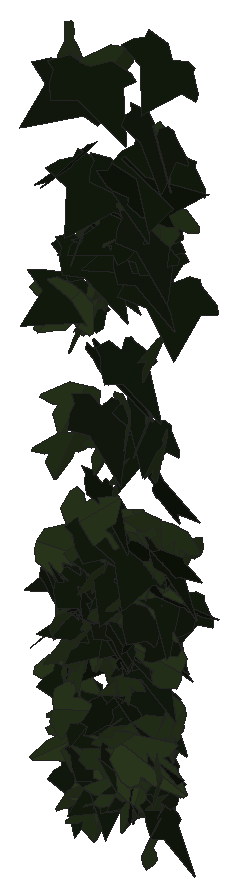
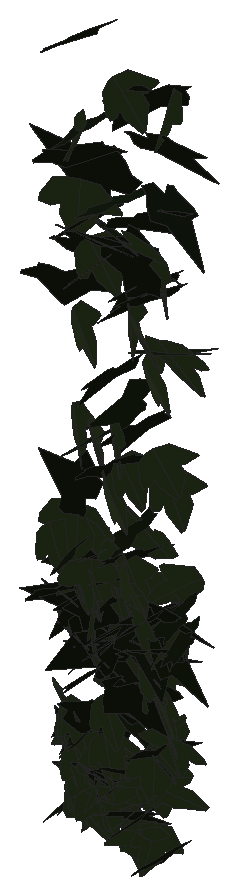
# SketchUp Ruby script. Lengths in inches.
U = 1.inch
M = Sketchup.active_model
def pt(a) = Geom::Point3d.new(a.map { |v| v * U })
def face(e, loops, mat)
  f = e.add_face(loops[0].map { |a| pt(a) })
  loops[1..].each { |l| e.add_face(l.map { |a| pt(a) }).erase! }
  f.material = f.back_material = mat if mat
  f
end
# faces: each face lists its corners as indices into pts; further lists are holes
def faces(e, pts, list, mat = nil) = list.each { |f| face(e, (f[0].is_a?(Array) ? f : [f]).map { |l| l.map { |i| pts[i] } }, mat) }
# xy, xz, yz: faces in a plane at the given z, y or x. An outline is a flat list of corners, or four numbers for a rectangle; further outlines are holes
def ring(l) = l.size == 4 ? [[l[0], l[1]], [l[2], l[1]], [l[2], l[3]], [l[0], l[3]]] : l.each_slice(2).to_a
def flat(e, list, mat, &to3) = list.each { |f| face(e, (f[0].is_a?(Array) ? f : [f]).map { |l| ring(l).map { |u, v| to3.(u, v) } }, mat) }
def xy(e, z, list, mat = nil) = flat(e, list, mat) { |x, y| [x, y, z] }
def xz(e, y, list, mat = nil) = flat(e, list, mat) { |x, z| [x, y, z] }
def yz(e, x, list, mat = nil) = flat(e, list, mat) { |y, z| [x, y, z] }
def lines(e, pts, list) = list.each { |a, b| e.add_line(pt(pts[a]), pt(pts[b])) }
# prism: a flat outline (further loops are holes) pulled along v
def prism(e, loops, v, mat = nil)
  f = face(e, loops, mat); d = Geom::Vector3d.new(v.map { |x| x * U })
  f.pushpull(f.normal.samedirection?(d) ? d.length : -d.length)
end
def box(e, o, s, mat = nil) = prism(e, [[o, [o[0] + s[0], o[1], o[2]], [o[0] + s[0], o[1] + s[1], o[2]], [o[0], o[1] + s[1], o[2]]]], [0, 0, s[2]], mat)
def at(x, y, z, deg = 0) = Geom::Transformation.translation(pt([x, y, z])) * Geom::Transformation.rotation(ORIGIN, Z_AXIS, deg.degrees)
def axes(o, x, y, z) = Geom::Transformation.new([*x, 0, *y, 0, *z, 0, *pt(o).to_a, 1])
def part(name) = M.definitions.add(name)
# library, detail: a bought-in or finely detailed component or shape, given as its bounding box
def library(name, o, s) = part(name).tap { |d| box(d.entities, o, s) }
def detail(e, o, s) = box(e.add_group.entities, o, s)
def put(e, d, t, mat = nil) = e.add_instance(d, t).tap { |i| i.material = mat if mat }
def group(e, t, mat = nil) = e.add_group.tap { |g| g.transformation = t; g.material = mat if mat }.entities
root = M.entities
M.materials.add("1026 AP 7946 SUNNY SIDE UP").color = [254, 231, 186]
M.materials.add("efeu1").color = [18, 25, 13]
M.materials.add("efeu2").color = [43, 57, 29]
c1 = part("ivyleaf_10")
p = [[0,0.5,-0.03],[-0.0625,2.02,-0.43],[-0.19,2.01,-0.46],[-0.54,1.05,-0.29],[-0.52,0.625,-0.18],[-0.83,0.76,-0.28],
  [-1.16,0.64,-0.33],[-1.15,0.33,-0.24],[-0.77,-0.39,0.02],[-0.3,-0.51,0.16],[0.04,-0.48,0.23],[-0.02,2.01,-0.4375],
  [-0.06,2.01,-0.43],[0.04,-0.49,0.23],[0.67,-0.49,0.14],[1.38,0.36,-0.2],[1.375,0.51,-0.24],[0.81,0.65,-0.19],
  [0.62,0.59,-0.15],[0.6,1.09,-0.28],[0.5,1.23,-0.31]]
faces(c1.entities,p,[[0,1,2,3,4,5,6,7,8,9,10],[11,12,0,13,14,15,16,17,18,19,20]],"efeu2")
c2 = part("ivyleaf_9")
p = [[1.54,2.16,1.25],[1.36,2.04,1.19],[-0.21,0.99,0.68],[-0.71,1.11,0.82],[-0.85,0.86,0.67],[-0.8,0.17,0.21],
  [-0.9,-0.01,0.1],[-0.67,-0.16,-0.02],[-0.08,-0.08,-0.05],[-0.03,-0.6,-0.4],[0.65,-0.88,-0.66],[0.83,-0.6,-0.49],
  [1.29,-0.42,-0.43],[1.8125,-0.07,-0.26],[1.21,0.44,0.15]]
faces(c2.entities,p,[[0,1,2,3,4,5,6,7,8,9,10,11,12,13,14]],"efeu1")
put(root,c1,axes([114.93,212.78,269.58],[0.41949,-0.00807,0.009],[0.01252,-0.02601,-0.27383],[0.01397,0.26566,-0.02496]),"1026 AP 7946 SUNNY SIDE UP")
put(root,c2,axes([114.86,212.53,271.03],[0.28826,-0.17994,-0.10556],[-0.0991,0.08044,-0.26386],[0.30931,0.19346,0.01384]),"1026 AP 7946 SUNNY SIDE UP")
put(root,c1,axes([115.09,212.77,270],[0.17426,-0.24249,-0.06948],[-0.06111,0.05481,-0.27406],[0.39044,0.1168,-0.01188]),"1026 AP 7946 SUNNY SIDE UP")
put(root,c1,axes([115.125,212.57,275.14],[0.43229,-0.08407,-0.10623],[-0.16878,-0.00212,-0.2944],[0.12262,0.29345,-0.03071]),"1026 AP 7946 SUNNY SIDE UP")
put(root,c1,axes([115.11,212.79,273.64],[-0.17544,-0.24056,0.1207],[0.00506,-0.12957,-0.26854],[0.42165,-0.09854,0.05344]),"1026 AP 7946 SUNNY SIDE UP")
put(root,c1,axes([115.03,212.61,278.78],[0.08865,-0.23721,-0.20622],[0.08034,0.20646,-0.23762],[0.48001,0.00925,0.07785]),"1026 AP 7946 SUNNY SIDE UP")
put(root,c2,axes([115.26,212.74,278.21],[-0.47065,-0.05058,0.01626],[-0.01884,-0.02524,-0.31199],[0.08129,-0.29868,0.0218]),"1026 AP 7946 SUNNY SIDE UP")
put(root,c2,axes([115.28,212.43,277.23],[-0.16105,0.28001,-0.03059],[0.00343,-0.03249,-0.30721],[-0.44302,-0.10205,0.00874]),"1026 AP 7946 SUNNY SIDE UP")
put(root,c1,axes([115.25,212.62,268.78],[0.1942,0.10053,-0.22778],[-0.29186,-0.1219,-0.1642],[-0.24758,0.22256,0.0149]),"1026 AP 7946 SUNNY SIDE UP")
put(root,c2,axes([115.22,212.72,275.13],[-0.38554,-0.12197,0.11628],[-0.03425,-0.17684,-0.24514],[0.25981,-0.20431,0.14024]),"1026 AP 7946 SUNNY SIDE UP")
put(root,c1,axes([115.18,212.5,273.13],[-0.14112,-0.27861,0.04935],[-0.01071,-0.04977,-0.30171],[0.44482,-0.08959,0.00839]),"1026 AP 7946 SUNNY SIDE UP")
put(root,c2,axes([115.05,212.93,267.92],[-0.06722,-0.24107,0.08265],[-0.01766,-0.08087,-0.25268],[0.39979,-0.04411,0.00273]),"1026 AP 7946 SUNNY SIDE UP")
put(root,c2,axes([114.93,212.54,271.35],[0.26419,-0.22109,-0.04019],[-0.04297,0.02665,-0.28586],[0.35005,0.17014,-0.00476]),"1026 AP 7946 SUNNY SIDE UP")
put(root,c2,axes([115.32,212.43,270.72],[-0.20392,0.2082,-0.12161],[0.06496,-0.11412,-0.25227],[-0.37161,-0.1342,0.02263]),"1026 AP 7946 SUNNY SIDE UP")
put(root,c1,axes([115.06,212.27,271.65],[0.05061,0.12629,0.26446],[0.09311,0.24905,-0.13279],[-0.43908,0.06737,0.00232]),"1026 AP 7946 SUNNY SIDE UP")
put(root,c2,axes([115.14,212.78,269.42],[-0.15404,-0.24708,0.01632],[0.00685,-0.02026,-0.27368],[0.3894,-0.09738,0.01127]),"1026 AP 7946 SUNNY SIDE UP")
put(root,c1,axes([115.22,212.82,274.88],[0.15842,-0.26962,0.06208],[0.01339,-0.0627,-0.29655],[0.43474,0.10018,-0.01349]),"1026 AP 7946 SUNNY SIDE UP")
put(root,c1,axes([115.28,212.51,269.99],[0.25029,-0.19239,-0.11752],[-0.08352,0.10212,-0.25564],[0.34074,0.16635,0.02366]),"1026 AP 7946 SUNNY SIDE UP")
put(root,c1,axes([115.26,212.71,269.17],[-0.26627,-0.20241,-0.0173],[0.02633,0.00637,-0.27169],[0.31813,-0.16994,0.00801]),"1026 AP 7946 SUNNY SIDE UP")
put(root,c1,axes([115.21,212.26,270.75],[-0.01818,-0.08253,-0.2877],[0.08763,0.27322,-0.08411],[0.44871,-0.0567,0.00477]),"1026 AP 7946 SUNNY SIDE UP")
put(root,c2,axes([115.54,212.63,271.34],[-0.42803,0.02994,0.05849],[-0.09319,-0.02411,-0.28059],[-0.03816,-0.27699,0.02909]),"1026 AP 7946 SUNNY SIDE UP")
put(root,c1,axes([115.36,212.48,276.22],[0.17653,-0.2613,-0.09098],[-0.02078,0.08854,-0.2916],[0.43246,0.11092,0.02312]),"1026 AP 7946 SUNNY SIDE UP")
put(root,c1,axes([115.32,212.61,268.05],[-0.15118,-0.22286,-0.11078],[0.0885,0.09125,-0.24908],[0.378,-0.1105,0.01401]),"1026 AP 7946 SUNNY SIDE UP")
put(root,c2,axes([115.47,212.55,270.84],[0.04089,0.26936,-0.00898],[-0.04255,-0.00763,-0.27752],[-0.4217,0.02689,0.02713]),"1026 AP 7946 SUNNY SIDE UP")
put(root,c1,axes([115.28,212.2,269.41],[0.03883,-0.11464,-0.26362],[0.18173,0.23753,-0.097],[0.40068,-0.09663,0.06954]),"1026 AP 7946 SUNNY SIDE UP")
put(root,c1,axes([115.41,212.33,270.33],[-0.14821,-0.25404,-0.09716],[0.05128,0.08696,-0.27864],[0.42221,-0.09974,-0.00026]),"1026 AP 7946 SUNNY SIDE UP")
put(root,c2,axes([115.55,212.67,270.13],[0.12324,0.15952,-0.2085],[-0.12133,-0.1883,-0.18397],[-0.38779,0.10961,-0.0087]),"1026 AP 7946 SUNNY SIDE UP")
put(root,c2,axes([115.68,212.72,270.5625],[-0.328,-0.06195,0.16458],[-0.19106,-0.12472,-0.21352],[0.19071,-0.2315,0.06915]),"1026 AP 7946 SUNNY SIDE UP")
put(root,c1,axes([115.18,212.83,276.52],[-0.16762,-0.00929,-0.29057],[0.36942,-0.16987,-0.08672],[-0.24569,-0.24907,0.06785]),"1026 AP 7946 SUNNY SIDE UP")
put(root,c1,axes([115.43,212.76,268.07],[0.2581,0.20013,-0.04493],[-0.0206,-0.04697,-0.26618],[-0.3218,0.16353,-0.019]),"1026 AP 7946 SUNNY SIDE UP")
put(root,c1,axes([115.43,212.76,275.31],[0.29729,-0.20461,0.10986],[0.0809,-0.09853,-0.28622],[0.35454,0.19406,-0.02681]),"1026 AP 7946 SUNNY SIDE UP")
put(root,c2,axes([115.34,212.65,268.58],[0.16106,-0.22662,-0.09419],[-0.03735,0.08804,-0.2553],[0.38167,0.10425,0.01476]),"1026 AP 7946 SUNNY SIDE UP")
put(root,c1,axes([115.5625,212.79,271.83],[0.0037,-0.28086,0.03917],[-0.00028,-0.03962,-0.28958],[0.44599,0.0023,-0.00051]),"1026 AP 7946 SUNNY SIDE UP")
put(root,c2,axes([115.29,212.66,275.9375],[0.14096,-0.25137,-0.15367],[0.0471,0.16169,-0.26373],[0.45604,0.061,0.07474]),"1026 AP 7946 SUNNY SIDE UP")
put(root,c1,axes([115.4,212.77,270.41],[0.37382,-0.1097,0.09198],[0.12465,-0.04274,-0.26993],[0.18493,0.25055,-0.00398]),"1026 AP 7946 SUNNY SIDE UP")
put(root,c2,axes([115.41,212.75,271.16],[-0.04881,-0.27369,0.06293],[-0.00309,-0.06281,-0.28408],[0.44147,-0.0307,0.00497]),"1026 AP 7946 SUNNY SIDE UP")
put(root,c2,axes([115.56,212.7,276.96],[-0.29439,-0.23287,0.05993],[-0.01984,-0.06579,-0.30656],[0.3774,-0.1851,0.03063]),"1026 AP 7946 SUNNY SIDE UP")
put(root,c1,axes([115.59,212.7,271.17],[0.31452,-0.18049,-0.07948],[-0.06424,0.06797,-0.27621],[0.30124,0.20294,0.02409]),"1026 AP 7946 SUNNY SIDE UP")
put(root,c2,axes([115.4,212.48,271.21],[0.03551,-0.24407,-0.1405],[0.01794,0.13613,-0.25079],[0.4382,0.01421,0.02166]),"1026 AP 7946 SUNNY SIDE UP")
put(root,c1,axes([115.64,212.51,267.94],[-0.14285,-0.25031,-0.01871],[0.02269,0.01256,-0.27409],[0.39382,-0.09152,0.00901]),"1026 AP 7946 SUNNY SIDE UP")
put(root,c1,axes([115.59,212.74,275.6],[0.11293,-0.28849,-0.03148],[0.06893,0.04026,-0.30131],[0.45065,0.06614,0.05397]),"1026 AP 7946 SUNNY SIDE UP")
put(root,c1,axes([115.38,212.54,268.69],[-0.21123,-0.05842,-0.22803],[0.34761,0.03211,-0.14698],[0.09158,-0.25664,0.03192]),"1026 AP 7946 SUNNY SIDE UP")
put(root,c2,axes([115.875,212.45,269.48],[-0.2352,0.22892,0.06602],[-0.06689,0.04715,-0.28127],[-0.36721,-0.15522,0.00895]),"1026 AP 7946 SUNNY SIDE UP")
put(root,c2,axes([115.44,212.58,275.99],[0.06549,-0.28884,-0.09893],[0.034,0.09785,-0.29806],[0.4766,0.03271,0.03486]),"1026 AP 7946 SUNNY SIDE UP")
put(root,c1,axes([115.69,212.74,273.29],[-0.04208,-0.27444,0.08002],[0.00642,-0.07994,-0.28429],[0.44911,-0.02457,0.01156]),"1026 AP 7946 SUNNY SIDE UP")
put(root,c1,axes([115.74,212.77,278.8],[-0.10948,-0.27775,0.11201],[-0.02523,-0.10962,-0.29544],[0.46924,-0.0707,0.01025]),"1026 AP 7946 SUNNY SIDE UP")
put(root,c2,axes([115.57,212.76,268.2],[-0.02878,-0.25262,0.07261],[-0.014,-0.07146,-0.26132],[0.41277,-0.02004,-0.0038]),"1026 AP 7946 SUNNY SIDE UP")
put(root,c1,axes([115.67,212.51,271.62],[-0.40683,-0.10944,-0.04361],[0.0781,-0.01094,-0.28791],[0.16677,-0.26184,0.02845]),"1026 AP 7946 SUNNY SIDE UP")
put(root,c2,axes([115.3,212.81,276.43],[0.17542,-0.00496,-0.29026],[0.43514,0.05895,0.11217],[0.08338,-0.29722,0.02529]),"1026 AP 7946 SUNNY SIDE UP")
put(root,c1,axes([115.73,212.47,271.46],[-0.02201,-0.2661,-0.09388],[0.01474,0.08924,-0.27396],[0.44127,-0.01625,0.00447]),"1026 AP 7946 SUNNY SIDE UP")
put(root,c2,axes([115.49,212.79,272.4375],[0.1315,-0.26089,0.07762],[0.02042,-0.07645,-0.28248],[0.42715,0.08397,-0.01039]),"1026 AP 7946 SUNNY SIDE UP")
put(root,c2,axes([115.53,212.4375,278.68],[-0.04491,-0.26333,-0.18299],[0.0668,0.17207,-0.2711],[0.49364,-0.04724,0.02004]),"1026 AP 7946 SUNNY SIDE UP")
put(root,c2,axes([115.47,212.75,274.37],[0.32076,-0.2051,-0.04694],[-0.02864,0.04438,-0.29716],[0.32872,0.20399,0.01992]),"1026 AP 7946 SUNNY SIDE UP")
put(root,c1,axes([115.45,212.4,272.09],[0.35817,-0.08196,-0.17884],[0.26975,-0.03239,0.24813],[-0.134,-0.28427,0.02147]),"1026 AP 7946 SUNNY SIDE UP")
put(root,c2,axes([115.87,212.66,270.63],[-0.39784,-0.09277,0.02579],[-0.02289,-0.03417,-0.27643],[0.14957,-0.252,0.02629]),"1026 AP 7946 SUNNY SIDE UP")
put(root,c2,axes([115.86,212.79,268.23],[-0.33661,-0.11831,0.10196],[-0.07977,-0.10703,-0.24381],[0.22977,-0.21048,0.06473]),"1026 AP 7946 SUNNY SIDE UP")
put(root,c1,axes([115.51,212.83,271.73],[0.23915,-0.05706,0.25343],[0.34876,-0.10791,-0.16746],[0.19089,0.26864,-0.01154]),"1026 AP 7946 SUNNY SIDE UP")
put(root,c2,axes([115.625,212.57,270.89],[0.13223,-0.26859,0.01094],[-0.00802,-0.01432,-0.28988],[0.42269,0.08375,-0.00893]),"1026 AP 7946 SUNNY SIDE UP")
put(root,c2,axes([115.72,212.77,268.91],[-0.17519,-0.23128,-0.06134],[0.1205,0.02615,-0.25789],[0.35513,-0.12296,0.05724]),"1026 AP 7946 SUNNY SIDE UP")
put(root,c1,axes([115.9,212.61,268.28],[-0.1383,-0.21603,0.12673],[-0.0209,-0.12749,-0.23883],[0.3913,-0.08317,0.03203]),"1026 AP 7946 SUNNY SIDE UP")
put(root,c1,axes([115.85,212.57,270.05],[-0.40292,0.09737,-0.02463],[0.02107,-0.03328,-0.28129],[-0.15645,-0.25525,0.02555]),"1026 AP 7946 SUNNY SIDE UP")
put(root,c2,axes([115.61,212.53,272.02],[0.13818,-0.23822,-0.15891],[0.06674,0.16938,-0.24574],[0.44007,0.04911,0.08717]),"1026 AP 7946 SUNNY SIDE UP")
put(root,c1,axes([115.78,212.52,268.73],[-0.35601,-0.07509,-0.10666],[0.1711,-0.00409,-0.24311],[0.10466,-0.24875,0.03461]),"1026 AP 7946 SUNNY SIDE UP")
put(root,c1,axes([115.89,212.78,272.9],[0.1088,-0.27306,0.05565],[0.02304,-0.05361,-0.29051],[0.43755,0.07072,0.00146]),"1026 AP 7946 SUNNY SIDE UP")
put(root,c2,axes([115.74,212.47,273.78],[0.00151,-0.29732,-0.06051],[-0.01785,0.05698,-0.30576],[0.4757,0.00308,-0.01128]),"1026 AP 7946 SUNNY SIDE UP")
put(root,c2,axes([116.16,212.51,276.51],[-0.42561,0.12949,-0.00205],[-0.03625,-0.05439,-0.3034],[-0.2004,-0.26517,0.05924]),"1026 AP 7946 SUNNY SIDE UP")
put(root,c1,axes([115.95,212.79,269.76],[-0.1104,-0.26402,0.02196],[0.00644,-0.02468,-0.28139],[0.41664,-0.06958,0.01017]),"1026 AP 7946 SUNNY SIDE UP")
put(root,c2,axes([115.85,212.91,273.36],[-0.15453,-0.26404,0.02867],[0.00006,-0.03129,-0.2902],[0.41772,-0.09767,0.01065]),"1026 AP 7946 SUNNY SIDE UP")
put(root,c1,axes([115.98,212.625,273.73],[0.2127,-0.20317,-0.16155],[-0.06119,0.1577,-0.24594],[0.39777,0.1329,0.04855]),"1026 AP 7946 SUNNY SIDE UP")
put(root,c1,axes([115.98,212.76,269.1875],[-0.12488,-0.25534,-0.00944],[0.00521,0.00705,-0.27544],[0.40165,-0.07948,0.00064]),"1026 AP 7946 SUNNY SIDE UP")
put(root,c1,axes([115.88,212.76,268.52],[0.32865,0.16156,-0.01929],[-0.00114,-0.03106,-0.2712],[-0.25591,0.20762,-0.02358]),"1026 AP 7946 SUNNY SIDE UP")
put(root,c2,axes([115.95,212.65,271.5],[-0.23666,-0.2353,0.02336],[-0.00264,-0.0274,-0.28758],[0.3719,-0.14993,0.01283]),"1026 AP 7946 SUNNY SIDE UP")
put(root,c1,axes([116.03,212.72,268.98],[-0.29337,-0.19053,0.01532],[0.00226,-0.02369,-0.27426],[0.30064,-0.18575,0.01701]),"1026 AP 7946 SUNNY SIDE UP")
put(root,c1,axes([115.95,212.375,271],[-0.17426,-0.22889,-0.12487],[0.10375,0.10109,-0.261],[0.39283,-0.12823,0.01354]),"1026 AP 7946 SUNNY SIDE UP")
put(root,c2,axes([115.61,212.6,270.44],[0.26033,-0.13659,0.17653],[0.26101,-0.06347,-0.21675],[0.2264,0.23024,0.0469]),"1026 AP 7946 SUNNY SIDE UP")
put(root,c1,axes([116.07,212.84,268.41],[-0.24861,-0.19558,0.07864],[-0.04434,-0.0763,-0.25827],[0.32778,-0.15866,0.02471]),"1026 AP 7946 SUNNY SIDE UP")
put(root,c2,axes([115.83,212.71,268.7],[0.09572,-0.25027,0.07398],[0.0087,-0.07395,-0.2655],[0.40993,0.06001,-0.01164]),"1026 AP 7946 SUNNY SIDE UP")
put(root,c2,axes([116.04,212.85,270.67],[-0.29814,-0.17383,0.10027],[0.00744,-0.13945,-0.2454],[0.31393,-0.16178,0.10104]),"1026 AP 7946 SUNNY SIDE UP")
put(root,c2,axes([115.89,212.69,270.89],[-0.01352,-0.27404,0.04044],[0.00562,-0.04093,-0.28265],[0.43561,-0.00797,0.0049]),"1026 AP 7946 SUNNY SIDE UP")
put(root,c2,axes([115.85,212.79,270.78],[0.08788,-0.27003,-0.02622],[0.00056,0.0245,-0.28389],[0.42626,0.05564,0.00578]),"1026 AP 7946 SUNNY SIDE UP")
put(root,c2,axes([115.87,212.57,270.84],[0.09003,-0.2599,-0.09076],[0.01483,0.09031,-0.2722],[0.43051,0.05124,0.02836]),"1026 AP 7946 SUNNY SIDE UP")
put(root,c2,axes([115.84,212.79,277.1],[-0.0022,-0.29756,0.04558],[0.11847,-0.04481,-0.297],[0.45836,0.01016,0.07698]),"1026 AP 7946 SUNNY SIDE UP")
put(root,c1,axes([116.29,212.58,271.85],[-0.3827,0.0759,0.13429],[-0.22322,-0.0339,-0.25376],[-0.07846,-0.2738,0.0669]),"1026 AP 7946 SUNNY SIDE UP")
put(root,c2,axes([115.9375,212.64,274.6],[0.11254,-0.2564,-0.12728],[-0.03859,0.11985,-0.27342],[0.44486,0.07526,0.00848]),"1026 AP 7946 SUNNY SIDE UP")
put(root,c1,axes([116.2,212.72,276.28],[-0.16013,-0.2691,0.09206],[-0.04487,-0.08638,-0.29689],[0.44435,-0.10569,0.0032]),"1026 AP 7946 SUNNY SIDE UP")
put(root,c1,axes([116.28,212.74,268.3],[-0.34216,-0.10141,0.1122],[-0.14064,-0.06635,-0.24682],[0.18785,-0.23439,0.01958]),"1026 AP 7946 SUNNY SIDE UP")
put(root,c1,axes([116.12,212.8,268.57],[-0.10068,0.24224,-0.08263],[-0.02033,-0.08707,-0.25638],[-0.40141,-0.05635,0.03371]),"1026 AP 7946 SUNNY SIDE UP")
put(root,c1,axes([116.2,212.81,271.66],[-0.36037,-0.15494,0.01778],[0.01545,-0.04651,-0.28165],[0.24481,-0.22515,0.04395]),"1026 AP 7946 SUNNY SIDE UP")
put(root,c1,axes([116.21,212.53,271.22],[-0.04537,-0.26962,0.01999],[0.00044,-0.02108,-0.27946],[0.42522,-0.02874,0.00242]),"1026 AP 7946 SUNNY SIDE UP")
put(root,c2,axes([116.01,212.49,270.69],[0.26713,-0.16624,-0.14855],[-0.1032,0.13438,-0.24005],[0.32927,0.17699,0.04528]),"1026 AP 7946 SUNNY SIDE UP")
put(root,c1,axes([116.2,212.75,273.63],[0.18337,-0.2653,-0.04693],[-0.0132,0.0444,-0.29811],[0.42266,0.11649,0.01105]),"1026 AP 7946 SUNNY SIDE UP")
put(root,c1,axes([116.23,212.77,271.02],[-0.1969,0.24712,-0.00286],[-0.09716,-0.03583,-0.276],[-0.37629,-0.12006,0.07276]),"1026 AP 7946 SUNNY SIDE UP")
put(root,c1,axes([116,212.75,272.125],[0.35405,-0.07561,0.14721],[0.20864,-0.05481,-0.24486],[0.14626,0.26122,-0.00704]),"1026 AP 7946 SUNNY SIDE UP")
put(root,c2,axes([116.23,212.48,268.11],[0.01843,-0.09506,0.25808],[0.12942,0.24047,0.09124],[-0.40178,0.0731,0.04123]),"1026 AP 7946 SUNNY SIDE UP")
put(root,c2,axes([116.58,212.66,276.375],[-0.38959,0.12192,0.12294],[-0.23561,-0.05715,-0.2622],[-0.12666,-0.2687,0.10958]),"1026 AP 7946 SUNNY SIDE UP")
put(root,c2,axes([116.46,212.78,268.66],[-0.40462,-0.00395,0.0617],[-0.09314,-0.02633,-0.26405],[0.01541,-0.26289,0.02397]),"1026 AP 7946 SUNNY SIDE UP")
put(root,c2,axes([116.17,212.44,270.3],[0.04141,-0.04363,0.2859],[0.22663,0.24164,0.02644],[-0.37962,0.1395,0.04697]),"1026 AP 7946 SUNNY SIDE UP")
put(root,c1,axes([116.31,212.78,268.68],[-0.14545,-0.24233,0.0529],[-0.01719,-0.05223,-0.26738],[0.38957,-0.09278,0.00795]),"1026 AP 7946 SUNNY SIDE UP")
put(root,c2,axes([116.52,212.73,276.32],[-0.43279,-0.05028,0.11206],[-0.15736,-0.05473,-0.2865],[0.10439,-0.29096,0.03271]),"1026 AP 7946 SUNNY SIDE UP")
put(root,c1,axes([116.29,212.72,271.53],[0.22791,-0.23892,-0.03909],[-0.00206,0.04189,-0.28687],[0.38005,0.1435,0.02189]),"1026 AP 7946 SUNNY SIDE UP")
put(root,c2,axes([116.0625,212.75,269.62],[-0.05192,-0.14789,-0.22898],[0.19284,0.1896,-0.14819],[0.37164,-0.11904,0.0449]),"1026 AP 7946 SUNNY SIDE UP")
put(root,c2,axes([116.1875,212.91,273.5625],[-0.0995,-0.25001,0.12131],[0.01648,-0.12432,-0.26367],[0.43519,-0.05245,0.03772]),"1026 AP 7946 SUNNY SIDE UP")
put(root,c1,axes([116.32,212.58,268.38],[-0.04483,-0.23434,0.14825],[0.02056,-0.14699,-0.24256],[0.43302,-0.01728,0.02686]),"1026 AP 7946 SUNNY SIDE UP")
put(root,c2,axes([116.24,212.58,271.8],[-0.13328,-0.25071,0.10393],[-0.00968,-0.10539,-0.27193],[0.42566,-0.0809,0.02636]),"1026 AP 7946 SUNNY SIDE UP")
put(root,c2,axes([116.07,212.72,270.65],[0.41959,-0.05233,0.01668],[0.01594,-0.0334,-0.27854],[0.08478,0.26526,-0.03015]),"1026 AP 7946 SUNNY SIDE UP")
put(root,c2,axes([116.48,212.78,270.59],[-0.40276,0.06671,-0.06711],[0.08208,-0.05652,-0.26983],[-0.12199,-0.25828,0.04003]),"1026 AP 7946 SUNNY SIDE UP")
put(root,c2,axes([116.15,212.8125,270.23],[0.09123,-0.26116,-0.05812],[0.00334,0.05666,-0.27489],[0.41962,0.05633,0.01482]),"1026 AP 7946 SUNNY SIDE UP")
put(root,c1,axes([116.32,212.42,268.43],[0.11737,0.18463,-0.2265],[0.05099,0.22137,0.20319],[0.44983,-0.07327,0.03607]),"1026 AP 7946 SUNNY SIDE UP")
put(root,c2,axes([116.51,212.74,268.61],[-0.41063,-0.01105,-0.00422],[0.00811,-0.02705,-0.26796],[0.01661,-0.25977,0.02655]),"1026 AP 7946 SUNNY SIDE UP")
put(root,c1,axes([116.42,212.8,268.88],[-0.11837,-0.25484,0.01914],[-0.00931,-0.01913,-0.27386],[0.40184,-0.07551,-0.00071]),"1026 AP 7946 SUNNY SIDE UP")
put(root,c2,axes([116.16,212.625,276.1],[0.14305,-0.28505,-0.06953],[-0.01149,0.06675,-0.30756],[0.45988,0.09033,0.01394]),"1026 AP 7946 SUNNY SIDE UP")
put(root,c2,axes([116.54,212.8,269],[-0.00509,-0.29693,0.03934],[0.00334,0.03985,0.30614],[-0.47107,0.00349,0.00175]),"1026 AP 7946 SUNNY SIDE UP")
put(root,c1,axes([116.54,212.65,271.27],[0.20678,0.12658,-0.20953],[-0.23966,-0.13586,-0.18876],[-0.29187,0.20124,0.00654]),"1026 AP 7946 SUNNY SIDE UP")
put(root,c1,axes([116.63,212.51,270.5],[0.10057,-0.00534,-0.28508],[-0.22773,0.24135,-0.03788],[0.37081,0.14967,0.05405]),"1026 AP 7946 SUNNY SIDE UP")
put(root,c1,axes([116.5,212.69,269.4],[-0.21735,-0.22287,0.02671],[-0.00487,-0.03004,-0.27001],[0.35301,-0.13764,0.01272]),"1026 AP 7946 SUNNY SIDE UP")
put(root,c2,axes([116.09,212.64,271.15],[0.29365,-0.04671,0.19832],[0.30831,0.00345,-0.1948],[0.04714,0.26838,0.03863]),"1026 AP 7946 SUNNY SIDE UP")
put(root,c1,axes([116.59,212.64,272.27],[-0.47188,-0.003,0.0261],[-0.0392,-0.02985,-0.30786],[0.00863,-0.29969,0.02863]),"1026 AP 7946 SUNNY SIDE UP")
put(root,c2,axes([116.87,212.5,270.88],[-0.2763,0.18598,0.16073],[-0.21436,0.08221,-0.26041],[-0.31454,-0.21939,0.03628]),"1026 AP 7946 SUNNY SIDE UP")
put(root,c2,axes([116.55,212.48,271.97],[0.33965,0.10681,-0.14037],[-0.18517,-0.07038,-0.24847],[-0.20058,0.24584,-0.00832]),"1026 AP 7946 SUNNY SIDE UP")
put(root,c1,axes([116.6,212.58,276.93],[-0.45769,-0.08064,0.01171],[-0.00958,-0.0222,-0.31062],[0.1278,-0.29047,0.01865]),"1026 AP 7946 SUNNY SIDE UP")
put(root,c1,axes([116.46,212.76,271.375],[0.23179,-0.21509,0.09156],[0.12183,-0.05535,-0.26707],[0.34585,0.16365,0.03272]),"1026 AP 7946 SUNNY SIDE UP")
put(root,c1,axes([116.59,212.65,268.33],[0.01489,-0.26481,0.01919],[-0.00405,-0.02023,-0.27308],[0.41757,0.00925,-0.00333]),"1026 AP 7946 SUNNY SIDE UP")
put(root,c2,axes([116.4,212.75,277.95],[-0.02709,-0.28051,0.11887],[0.03399,-0.118,-0.28892],[0.47669,-0.00753,0.02736]),"1026 AP 7946 SUNNY SIDE UP")
put(root,c2,axes([116.41,212.58,276.61],[0.01373,-0.30123,-0.01471],[0.00781,0.01272,-0.31033],[0.474,0.00851,0.00554]),"1026 AP 7946 SUNNY SIDE UP")
put(root,c1,axes([116.6,212.54,275.04],[0.08212,-0.29089,0.02705],[0.0028,-0.02803,-0.30461],[0.45949,0.05216,-0.00298]),"1026 AP 7946 SUNNY SIDE UP")
put(root,c2,axes([116.42,212.54,271.1],[0.06813,-0.23027,-0.1845],[-0.03847,0.17622,-0.24025],[0.45581,0.04929,0.0073]),"1026 AP 7946 SUNNY SIDE UP")
put(root,c1,axes([116.51,212.67,277.9],[-0.13577,0.28085,-0.0793],[0.03911,-0.07455,-0.30312],[-0.45689,-0.08984,-0.00239]),"1026 AP 7946 SUNNY SIDE UP")
put(root,c2,axes([116.24,212.44,277.07],[0.01409,-0.00316,0.32108],[0.42456,-0.15573,-0.01053],[0.2449,0.27015,-0.00021]),"1026 AP 7946 SUNNY SIDE UP")
put(root,c2,axes([116.36,212.65,268.73],[-0.01815,-0.09273,0.26459],[0.22866,-0.22027,-0.07632],[0.36434,0.13362,0.06108]),"1026 AP 7946 SUNNY SIDE UP")
put(root,c2,axes([116.3125,212.83,272.73],[0.13574,-0.1129,0.27177],[0.18749,-0.23719,-0.14581],[0.41142,0.14534,-0.02322]),"1026 AP 7946 SUNNY SIDE UP")
put(root,c1,axes([116.72,212.18,267.85],[0.07806,-0.05568,0.28924],[-0.20573,0.24939,0.07615],[-0.40085,-0.13884,0.01724]),"1026 AP 7946 SUNNY SIDE UP")
put(root,c2,axes([116.61,212.71,277.57],[-0.25367,-0.26316,-0.01229],[0.02295,0.00328,-0.31778],[0.41348,-0.16163,0.0101]),"1026 AP 7946 SUNNY SIDE UP")
put(root,c1,axes([116.99,212.3125,270.55],[0.02622,0.09298,0.28045],[-0.4491,0.03368,0.00638],[-0.04698,-0.27012,0.09554]),"1026 AP 7946 SUNNY SIDE UP")
put(root,c1,axes([116.71,212.45,273.56],[0.09191,-0.28417,-0.07483],[0.00592,0.07315,-0.29788],[0.46053,0.05577,0.01876]),"1026 AP 7946 SUNNY SIDE UP")
put(root,c1,axes([116.65,212.78,269.45],[0.04481,-0.25882,0.04754],[0.11624,-0.03809,-0.25911],[0.39714,0.04036,0.07048]),"1026 AP 7946 SUNNY SIDE UP")
put(root,c1,axes([116.42,212.28,269.09],[0.21338,0.1484,0.23348],[0.28525,0.13722,-0.20442],[-0.31486,0.22488,-0.02697]),"1026 AP 7946 SUNNY SIDE UP")
put(root,c2,axes([116.5,212.76,271.86],[0.18059,-0.25151,0.0236],[0.00003,-0.02672,-0.28477],[0.39732,0.11432,-0.0107]),"1026 AP 7946 SUNNY SIDE UP")
put(root,c1,axes([116.77,212.3,268.84],[0.01768,-0.07562,-0.28157],[-0.01449,0.27286,-0.07669],[0.44502,0.01189,0.00869]),"1026 AP 7946 SUNNY SIDE UP")
put(root,c1,axes([116.79,212.83,271.99],[-0.12086,-0.26901,0.03788],[0.00305,-0.04034,-0.28815],[0.42724,-0.07581,0.01277]),"1026 AP 7946 SUNNY SIDE UP")
put(root,c1,axes([116.76,212.7,269.61],[0.26453,-0.20935,-0.01548],[-0.0312,0.00177,-0.27627],[0.32841,0.16879,-0.01378]),"1026 AP 7946 SUNNY SIDE UP")
put(root,c2,axes([116.72,212.63,279.12],[-0.19342,-0.24883,0.13812],[-0.03048,-0.13997,-0.28377],[0.44446,-0.11788,0.04065]),"1026 AP 7946 SUNNY SIDE UP")
put(root,c2,axes([116.7,212.85,271.24],[-0.18648,-0.25116,0.01253],[0.01703,-0.02011,-0.28563],[0.39513,-0.11766,0.01822]),"1026 AP 7946 SUNNY SIDE UP")
put(root,c2,axes([116.59,212.54,268.22],[0.1959,-0.22814,-0.07921],[-0.0608,0.06501,-0.2674],[0.37298,0.13042,-0.00198]),"1026 AP 7946 SUNNY SIDE UP")
put(root,c2,axes([116.67,212.74,275.79],[-0.28234,-0.21694,-0.12593],[0.15992,0.07201,-0.28807],[0.35635,-0.2042,0.0295]),"1026 AP 7946 SUNNY SIDE UP")
